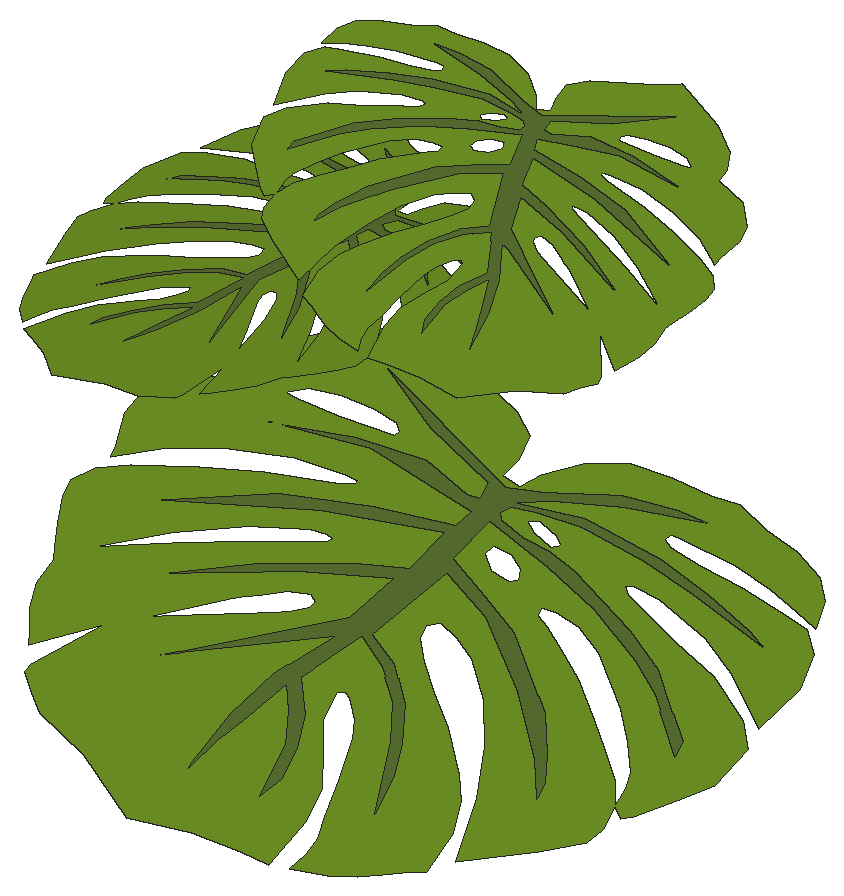
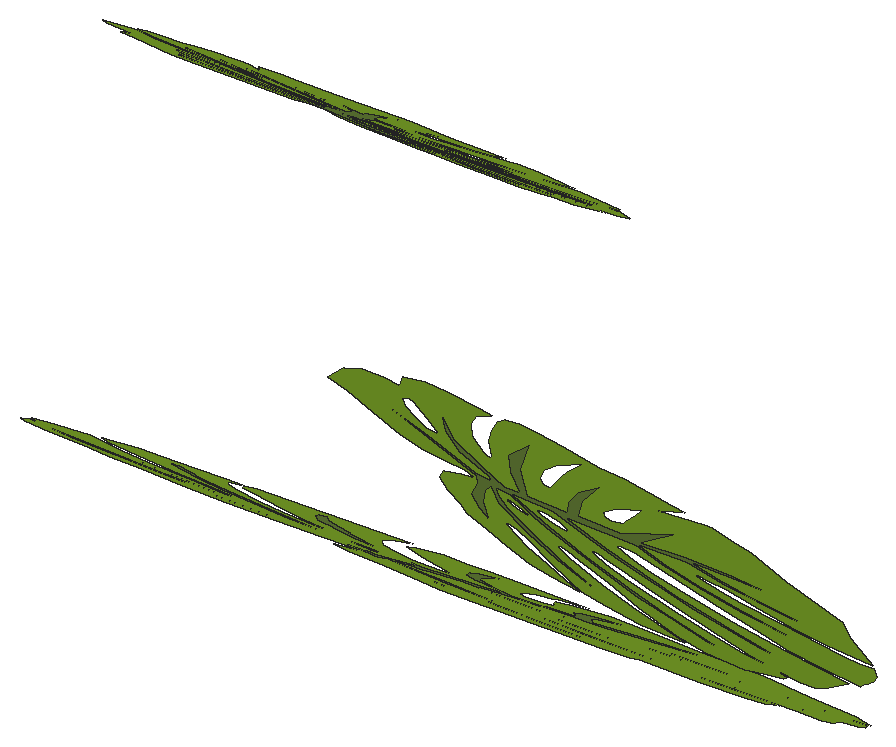
# SketchUp Ruby script. Lengths in inches.
U = 1.inch
M = Sketchup.active_model
def pt(a) = Geom::Point3d.new(a.map { |v| v * U })
def face(e, loops, mat)
  f = e.add_face(loops[0].map { |a| pt(a) })
  loops[1..].each { |l| e.add_face(l.map { |a| pt(a) }).erase! }
  f.material = f.back_material = mat if mat
  f
end
# faces: each face lists its corners as indices into pts; further lists are holes
def faces(e, pts, list, mat = nil) = list.each { |f| face(e, (f[0].is_a?(Array) ? f : [f]).map { |l| l.map { |i| pts[i] } }, mat) }
# xy, xz, yz: faces in a plane at the given z, y or x. An outline is a flat list of corners, or four numbers for a rectangle; further outlines are holes
def ring(l) = l.size == 4 ? [[l[0], l[1]], [l[2], l[1]], [l[2], l[3]], [l[0], l[3]]] : l.each_slice(2).to_a
def flat(e, list, mat, &to3) = list.each { |f| face(e, (f[0].is_a?(Array) ? f : [f]).map { |l| ring(l).map { |u, v| to3.(u, v) } }, mat) }
def xy(e, z, list, mat = nil) = flat(e, list, mat) { |x, y| [x, y, z] }
def xz(e, y, list, mat = nil) = flat(e, list, mat) { |x, z| [x, y, z] }
def yz(e, x, list, mat = nil) = flat(e, list, mat) { |y, z| [x, y, z] }
def lines(e, pts, list) = list.each { |a, b| e.add_line(pt(pts[a]), pt(pts[b])) }
# prism: a flat outline (further loops are holes) pulled along v
def prism(e, loops, v, mat = nil)
  f = face(e, loops, mat); d = Geom::Vector3d.new(v.map { |x| x * U })
  f.pushpull(f.normal.samedirection?(d) ? d.length : -d.length)
end
def box(e, o, s, mat = nil) = prism(e, [[o, [o[0] + s[0], o[1], o[2]], [o[0] + s[0], o[1] + s[1], o[2]], [o[0], o[1] + s[1], o[2]]]], [0, 0, s[2]], mat)
def at(x, y, z, deg = 0) = Geom::Transformation.translation(pt([x, y, z])) * Geom::Transformation.rotation(ORIGIN, Z_AXIS, deg.degrees)
def axes(o, x, y, z) = Geom::Transformation.new([*x, 0, *y, 0, *z, 0, *pt(o).to_a, 1])
def part(name) = M.definitions.add(name)
# library, detail: a bought-in or finely detailed component or shape, given as its bounding box
def library(name, o, s) = part(name).tap { |d| box(d.entities, o, s) }
def detail(e, o, s) = box(e.add_group.entities, o, s)
def put(e, d, t, mat = nil) = e.add_instance(d, t).tap { |i| i.material = mat if mat }
def group(e, t, mat = nil) = e.add_group.tap { |g| g.transformation = t; g.material = mat if mat }.entities
root = M.entities
M.materials.add("[0059_DarkOliveGreen]").color = [85, 107, 47]
M.materials.add("[0061_OliveDrab]").color = [107, 142, 35]
p = [[520.239,153.728,22.334],[520.977,153.593,22.249],[521.408,154.12,22.583],[522.47,154.844,23.043],[523.928,155.29,23.326],[525.483,155.364,23.372],
  [527.043,155.298,23.331],[528.141,155.35,23.364],[529.435,154.984,23.132],[530.862,154.714,22.96],[532.104,154.265,22.675],[532.723,153.723,22.331],
  [533.025,152.934,21.83],[532.093,153.181,21.987],[530.828,153.488,22.182],[529.252,153.745,22.345],[527.011,153.899,22.443],[526.638,153.881,22.431],
  [526.532,153.708,22.322],[526.902,153.559,22.227],[528.159,153.379,22.113],[529.904,153.234,22.021],[532.065,152.927,21.826],[532.759,152.811,21.753],
  [533.5,152.24,21.39],[533.766,151.206,20.734],[533.323,149.779,19.828],[531.296,150.951,20.572],[529.832,151.573,20.967],[527.617,152.106,21.305],
  [526.505,152.213,21.373],[526.248,152.109,21.307],[526.529,151.906,21.178],[527.285,151.694,21.044],[528.944,151.172,20.712],[530.863,150.663,20.389],
  [532.636,149.846,19.871],[533.406,149.141,19.423],[533.12,147.885,18.626],[532.28,147.119,18.14],[531.289,146.285,17.61],[530.906,146.106,17.497],
  [530.469,146.351,17.652],[530.45,146.926,18.017],[530.274,147.368,18.298],[529.562,148.138,18.787],[528.645,148.933,19.291],[526.842,150.145,20.06],
  [525.69,150.597,20.347],[524.704,150.736,20.435],[524.157,150.71,20.419],[524.197,150.465,20.263],[524.687,150.278,20.145],[525.582,149.835,19.864],
  [526.719,149.264,19.502],[528.052,148.375,18.937],[528.935,147.761,18.547],[529.953,147.029,18.083],[530.587,145.623,17.19],[530.336,145.135,16.881],
  [529.048,144.431,16.434],[526.716,143.335,15.738],[526.091,145.152,16.891],[525.239,146.591,17.805],[524.247,147.765,18.55],[523.042,148.695,19.14],
  [522.129,149.096,19.394],[521.358,149.33,19.543],[520.964,149.078,19.383],[521.028,148.686,19.134],[521.632,148.134,18.784],[522.555,147.456,18.354],
  [523.711,146.693,17.869],[525.038,145.584,17.166],[525.645,144.928,16.749],[526.0625,144.019,16.173],[526.027,142.793,15.394],[525.311,142.526,15.225],
  [524.754,142.268,15.061],[524,141.974,14.875],[523.069,141.698,14.7],[521.757,141.5,14.574],[521.958,141.994,14.888],[522.013,142.537,15.232],
  [521.76,143.172,15.635],[521.467,144.232,16.308],[521.038,145.456,17.084],[520.687,145.968,17.409],[520.114,146.479,17.734],[519.797,146.582,17.799],
  [519.588,146.465,17.725],[519.651,146.076,17.478],[519.728,145.601,17.176],[520.331,144.878,16.718],[521.117,143.818,16.045],[521.274,142.853,15.432],
  [521.048,141.374,14.494],[519.906,141.415,14.52],[518.002,141.406,14.514],[515.688,141.161,14.358],[513.072,142.342,15.108],[510.856,142.96,15.5],
  [510.215,143.416,15.79],[509.573,143.871,16.079],[509.617,144.147,16.254],[511.051,145.867,17.346],[509.885,145.112,16.866],[509.122,144.609,16.547],
  [508.903,144.952,16.765],[508.417,145.561,17.151],[508.134,146.268,17.6],[508.149,147.035,18.087],[507.939,147.365,18.296],[507.535,148.016,18.709],
  [507.135,148.747,19.173],[507.041,149.268,19.504],[507.566,149.822,19.855],[508.582,150.238,20.119],[510.698,150.89,20.533],[512.804,151.417,20.868],
  [515.421,151.879,21.161],[515.892,152.019,21.249],[515.876,152.12,21.314],[515.397,152.167,21.344],[513.461,152.076,21.286],[511.296,151.658,21.02],
  [509.326,151.059,20.64],[507.788,150.253,20.129],[507.731,150.604,20.352],[507.321,151.534,20.942],[507.475,152.24,21.39],[508.405,153.114,21.944],
  [510.241,153.597,22.251],[510.156,154.121,22.584],[510.574,154.859,23.052],[512.01,155.715,23.595],[514.962,156.822,24.298],[515.988,156.441,24.056],
  [517.607,155.999,23.776],[519.337,155.496,23.457],[520.273,155.004,23.144],[520.39,154.282,22.686],[518.431,148.552,19.049],[513.403,145.677,17.225],
  [518.35,147.893,18.631],[517.287,146.364,17.661],[516.782,144.862,16.707],[516.578,143.22,15.666],[516.566,143.072,15.571],[516.917,144.063,16.2],
  [517.257,144.808,16.673],[517.863,146.206,17.561],[518.468,145.532,17.133],[519.09,144.616,16.551],[519.342,143.064,15.566],[519.667,143.697,15.968],
  [519.517,144.624,16.556],[519.048,145.592,17.171],[518.197,146.488,17.739],[519.216,148.156,18.798],[520.445,147.601,18.446],[521.489,146.808,17.943],
  [522.275,145.764,17.28],[523.251,143.743,15.997],[523.066,144.883,16.721],[522.672,145.793,17.299],[521.912,146.866,17.98],[520.801,147.799,18.571],
  [519.496,148.335,18.911],[520.527,150.634,20.37],[522.592,149.906,19.909],[525.25,148.244,18.854],[527.034,146.778,17.923],[527.919,145.773,17.285],
  [527.845,146.229,17.575],[527.318,146.995,18.061],[526.387,148.058,18.736],[523.821,149.814,19.85],[522.208,150.444,20.25],[520.453,151.089,20.659],
  [520.797,152.4,21.491],[523.497,151.81,21.117],[525.806,151.181,20.718],[528.099,150.283,20.148],[529.398,149.627,19.732],[531.307,148.244,18.854],
  [531.235,148.688,19.135],[530.237,149.4,19.588],[529.041,150.3,20.159],[527.361,151.03,20.622],[524.41,151.986,21.228],[523.279,152.252,21.397],
  [522.101,152.349,21.459],[521.116,152.555,21.59],[520.9375,152.74,21.707],[521.184,152.971,21.854],[522.031,153.084,21.926],[523.749,153.165,21.977],
  [526.337,152.908,21.814],[528.506,152.571,21.6],[531.943,151.882,21.162],[531.023,152.218,21.376],[528.97,152.759,21.72],[526.8,153.184,21.989],
  [523.632,153.454,22.16],[521.277,153.163,21.976],[522.379,153.559,22.227],[524.638,154.099,22.57],[527.701,154.565,22.865],[526.307,154.596,22.885],
  [524.315,154.412,22.769],[521.829,153.719,22.329],[520.565,153.457,22.162],[514.225,155.41,23.402],[517.013,154.195,22.631],[519.922,153.378,22.112],
  [519.998,152.906,21.8125],[519.516,152.883,21.798],[517.587,153.351,22.095],[514.937,153.226,22.015],[511.951,152.729,21.7],[515.647,153.069,21.916],
  [518.13,152.723,21.696],[520.003,152.467,21.534],[519.793,151.994,21.234],[516.853,151.63,21.003],[513.708,151.027,20.62],[509.929,149.559,19.688],
  [515.374,150.972,20.585],[519.597,151.665,21.025],[519.278,150.415,20.231],[517.501,149.997,19.967],[514.48,149.005,19.337],[511.591,147.71,18.515],
  [515.962,149.211,19.467],[518.978,149.955,19.94],[513.428,149.857,19.877],[512.041,149.289,19.517],[511.268,148.972,19.316],[508.928,147.683,18.498],
  [509.849,148.025,18.715],[511.774,148.772,19.189],[513.71,149.419,19.6],[515.474,150,19.968],[516.209,150.245,20.124],[516.298,150.385,20.213],
  [516.027,150.448,20.253],[515.398,150.397,20.22],[515.212,148.223,18.841],[514.812,148.039,18.724],[514.426,147.862,18.611],[512.179,146.515,17.757],
  [514.023,147.177,18.177],[516.004,147.898,18.634],[516.507,148.072,18.745],[516.998,148.382,18.941],[517.074,148.601,19.08],[516.762,148.742,19.17],
  [515.998,148.585,19.07],[514.252,154.151,22.603],[513.588,154.164,22.611],[512.464,154.008,22.512],[511.82,153.664,22.294],[512.246,153.608,22.258],
  [514.006,153.588,22.245],[516.113,153.638,22.277],[516.179,153.794,22.376],[515.888,153.999,22.507],[514.916,154.137,22.594],[521.268,151.538,20.944],
  [521.805,151.154,20.701],[522.596,151.038,20.627],[522.907,151.174,20.713],[522.71,151.51,20.926],[522.132,151.777,21.096],[521.398,151.832,21.131],
  [522.852,152.786,21.736],[522.311,152.913,21.817],[521.917,152.787,21.737],[522.368,152.557,21.591],[523.188,152.358,21.465],[523.484,152.509,21.56],
  [523.074,152.733,21.703],[518.622,156.433,29.335],[519.41,156.337,29.494],[519.887,155.03,29.031],[519.861,154.246,28.672],[519.455,153.79,28.363],
  [518.989,153.568,28.144],[519.453,152.851,27.941],[519.176,152.194,27.575],[518.673,151.824,27.28],[517.725,151.5,26.89],[517.413,151.351,26.743],
  [517.351,152.139,27.081],[516.919,152.946,27.332],[516.249,153.72,27.507],[515.42,154.281,27.545],[515.157,154.387,27.525],[515.067,154.344,27.483],
  [515.174,154.152,27.424],[516.019,153.237,27.231],[516.573,152.427,27.01],[517.03,151.556,26.737],[517.165,151.09,26.5625],[516.96,150.691,26.331],
  [516.492,150.473,26.112],[515.71,150.239,25.806],[514.992,150.044,25.534],[514.626,149.946,25.395],[514.008,149.583,25.074],[513.301,149.33,24.778],
  [512.579,149.175,24.523],[512.198,149.074,24.379],[512.251,149.513,24.59],[512.321,150.178,24.906],[511.59,148.991,24.186],[511.386,148.85,24.07],
  [510.716,148.809,23.879],[510.046,148.768,23.688],[508.51,149.073,23.43],[506.327,149.222,22.935],[505.447,149.956,23.038],[504.565,150.469,23.041],
  [503.999,150.756,23.024],[505.097,151.507,23.643],[505.956,151.915,24.048],[507.185,152.199,24.492],[508.055,152.375,24.794],[508.477,152.577,24.993],
  [508.823,152.741,25.156],[508.821,152.852,25.206],[508.589,152.889,25.162],[507.906,152.803,24.948],[507.326,152.658,24.734],[506.13,152.202,24.221],
  [505.13,151.786,23.777],[504.495,151.557,23.511],[504.079,151.289,23.284],[503.771,151.005,23.077],[503.32,151.448,23.16],[503.11,151.827,23.275],
  [502.997,152.165,23.398],[502.946,152.435,23.506],[502.83,152.751,23.618],[503.811,153.333,24.132],[504.746,153.645,24.513],[505.563,153.789,24.787],
  [507.085,153.951,25.252],[508.245,153.998,25.572],[509.227,154.067,25.855],[509.959,154.163,26.087],[510.307,154.329,26.251],[510.329,154.552,26.357],
  [509.778,154.649,26.258],[509.026,154.706,26.09],[507.707,154.595,25.701],[506.289,154.313,25.209],[504.72,153.869,24.606],[502.949,153.188,23.845],
  [502.753,154.324,24.304],[502.725,154.997,24.599],[503.004,155.292,24.804],[503.652,155.6,25.109],[504.445,155.779,25.393],[505.516,155.848,25.699],
  [506.427,155.898,25.957],[507.773,155.956,26.329],[508.768,155.919,26.568],[509.547,155.885,26.754],[509.927,155.842,26.832],[510.145,155.945,26.935],
  [509.911,156.104,26.945],[509.338,156.303,26.887],[508.432,156.4,26.698],[506.605,156.317,26.19],[505.53,156.192,25.857],[504.571,156.023,25.535],
  [504.129,155.863,25.349],[503.249,155.603,25.006],[503.216,155.789,25.081],[503.433,156.444,25.431],[503.663,157.026,25.751],[504.552,157.688,26.277],
  [505.485,157.811,26.573],[506.977,157.718,26.915],[508.288,157.442,27.128],[509.487,157.242,27.347],[510.012,157.138,27.435],[510.308,157.158,27.52],
  [510.273,157.275,27.564],[509.666,157.523,27.519],[508.199,157.867,27.296],[507.01,157.969,27.036],[505.11,157.964,26.544],[506.065,158.749,27.142],
  [507.03,159.16,27.576],[507.841,159.228,27.815],[508.259,159.096,27.863],[509.518,158.662,27.992],[510.449,158.262,28.052],[511.183,158.01,28.128],
  [511.477,157.98,28.19],[511.568,158.089,28.263],[511.408,158.197,28.27],[510.237,158.725,28.206],[509.293,159.027,28.098],[508.453,159.223,27.97],
  [507.816,159.356,27.866],[508.599,159.644,28.196],[509.33,159.731,28.424],[510.275,159.608,28.612],[511.16,159.353,28.725],[512.062,159.177,28.878],
  [512.532,158.859,28.856],[513.313,158.472,28.884],[513.979,158.022,28.853],[514.297,157.423,28.666],[514.203,156.801,28.363],[513.975,156.44,28.142],
  [514.429,156.305,28.199],[514.811,156.604,28.431],[515.452,156.91,28.733],[516.29,156.889,28.939],[517.506,156.66,29.15],[516.315,155.66,28.394],
  [518.605,155.481,28.903],[517.134,155.734,28.639],[514.057,156.266,28.085],[513.681,156.726,28.195],[513.085,157.715,28.485],[512.304,158.334,28.562],
  [511.628,158.693,28.549],[512.679,157.656,28.354],[513.293,156.799,28.128],[513.486,156.319,27.962],[512.623,157.085,28.084],[510.925,157.807,27.971],
  [509.567,158.19,27.793],[508.168,158.487,27.566],[507.465,158.576,27.425],[509.63,157.978,27.714],[510.917,157.555,27.855],[512.334,156.982,27.963],
  [513.07,156.484,27.929],[513.373,156.205,27.882],[513.3,156.031,27.785],[513.066,155.993,27.708],[512.439,156.16,27.621],[511.81,156.43,27.58],
  [511.065,156.608,27.469],[508.911,156.952,27.069],[507.532,157.061,26.763],[506.242,156.961,26.386],[505.197,156.896,26.087],[504.801,156.708,25.901],
  [506.818,156.843,26.481],[507.958,156.801,26.756],[509.759,156.606,27.132],[511.349,156.282,27.395],[513.089,155.835,27.642],[512.182,155.131,27.093],
  [510.838,155.299,26.823],[509.573,155.437,26.559],[506.947,155.305,25.824],[505.647,155.058,25.379],[504.778,154.841,25.058],[504.372,154.648,24.866],
  [505.603,154.88,25.287],[507.628,155.087,25.902],[510.222,155.151,26.598],[511.777,154.938,26.903],[510.388,153.589,25.94],[509.342,153.688,25.715],
  [508.065,153.55,25.325],[506.837,153.253,24.875],[505.912,152.934,24.494],[504.898,152.451,24.016],[506.999,153.133,24.863],[508.215,153.41,25.3],
  [509.348,153.501,25.632],[510.373,153.431,25.865],[509.491,152.38,25.166],[508.364,152.189,24.791],[507.358,151.863,24.385],[506.534,151.471,23.997],
  [506.17,151.088,23.732],[507.551,151.745,24.382],[508.586,152.006,24.766],[509.417,152.159,25.048],[508.5625,151.344,24.462],[508.115,150.905,24.15],
  [507.472,150.349,23.735],[507.588,150.421,23.797],[508.828,151.242,24.485],[509.815,152.078,25.114],[510.563,153.076,25.754],[511.068,150.718,24.826],
  [511.062,153.405,26.031],[511.948,154.207,26.618],[512.75,153.052,26.306],[513.569,151.182,25.678],[513.274,152.56,26.221],[512.672,153.831,26.636],
  [512.182,154.502,26.811],[513.051,155.17,27.334],[514.458,153.717,27.044],[515.849,151.6,26.452],[515.279,153.297,27.067],[514.303,154.42,27.32],
  [513.227,155.376,27.472],[513.514,155.653,27.67],[514.596,155.272,27.778],[516.037,154.768,27.923],[517.485,153.62,27.78],[516.495,154.652,27.988],
  [515.36,155.419,28.041],[514.08,155.717,27.845],[513.873,155.857,27.854],[514.293,156.057,28.052],[514.458,152.675,26.577],[513.978,153.455,26.803],
  [513.726,153.647,26.825],[513.549,153.69,26.799],[513.477,153.601,26.74],[513.62,153.29,26.637],[513.97,152.547,26.394],[514.347,151.726,26.123],
  [514.638,150.863,25.81],[514.789,150.457,25.667],[514.746,151.685,26.207],[512.224,152.77,26.044],[511.995,153.047,26.11],[511.735,153.065,26.051],
  [511.592,152.942,25.959],[511.569,152.667,25.83],[511.662,152.451,25.757],[512,151.584,25.455],[512.322,150.782,25.177],[512.369,152.012,25.741],
  [517.889,154.729,28.381],[517.247,155.071,28.37],[516.681,155.267,28.3125],[516.378,155.249,28.226],[516.282,155.159,28.161],[517.225,154.572,28.14],
  [518.0625,154.11,28.148],[518.307,154.022,28.172],[518.286,154.355,28.316],[511.958,155.901,27.381],[511.472,155.931,27.27],[511.106,155.827,27.129],
  [511.14,155.68,27.072],[511.604,155.523,27.12],[512.167,155.558,27.281],[512.346,155.73,27.404],[512.8,156.479,27.857],[512.297,156.6,27.782],
  [511.923,156.605,27.688],[511.939,156.455,27.625],[512.483,156.328,27.708],[512.88,156.315,27.804],[522.447,153.259,35.965],[521.96,153.17,35.909],
  [521.675,153.517,36.129],[520.974,153.996,36.433],[520.012,154.29,36.62],[518.986,154.338,36.65],[517.956,154.295,36.623],[517.232,154.329,36.645],
  [516.377,154.088,36.491],[515.436,153.91,36.378],[514.616,153.613,36.19],[514.207,153.255,35.963],[514.008,152.734,35.632],[514.623,152.898,35.736],
  [515.458,153.1,35.865],[516.498,153.27,35.972],[517.977,153.371,36.037],[518.224,153.36,36.029],[518.293,153.245,35.957],[518.049,153.147,35.895],
  [517.22,153.028,35.819],[516.068,152.933,35.759],[514.642,152.73,35.63],[514.184,152.654,35.581],[513.694,152.277,35.342],[513.519,151.594,34.909],
  [513.812,150.652,34.311],[515.149,151.426,34.802],[516.115,151.836,35.0625],[517.577,152.188,35.286],[518.311,152.259,35.331],[518.481,152.19,35.287],
  [518.296,152.056,35.202],[517.797,151.917,35.113],[516.702,151.572,34.895],[515.435,151.236,34.681],[514.265,150.697,34.339],[513.757,150.231,34.044],
  [513.945,149.402,33.518],[514.5,148.897,33.197],[515.154,148.346,32.847],[515.407,148.228,32.773],[515.695,148.39,32.875],[515.708,148.769,33.116],
  [515.823,149.061,33.301],[516.294,149.57,33.624],[516.899,150.094,33.957],[518.089,150.894,34.464],[518.849,151.192,34.654],[519.5,151.284,34.712],
  [519.861,151.267,34.701],[519.834,151.105,34.598],[519.511,150.982,34.52],[518.92,150.69,34.335],[518.17,150.313,34.096],[517.29,149.726,33.723],
  [516.707,149.321,33.466],[516.036,148.837,33.159],[515.617,147.909,32.57],[515.783,147.587,32.366],[516.633,147.123,32.071],[518.172,146.399,31.612],
  [518.584,147.599,32.373],[519.147,148.548,32.976],[519.802,149.323,33.468],[520.597,149.937,33.857],[521.199,150.201,34.025],[521.708,150.356,34.123],
  [521.968,150.189,34.017],[521.926,149.931,33.853],[521.528,149.567,33.622],[520.918,149.12,33.338],[520.156,148.616,33.018],[519.28,147.884,32.554],
  [518.879,147.451,32.279],[518.603,146.851,31.899],[518.627,146.041,31.385],[519.099,145.865,31.273],[519.467,145.695,31.165],[519.964,145.501,31.042],
  [520.579,145.319,30.926],[521.445,145.188,30.843],[521.312,145.514,31.05],[521.276,145.873,31.278],[521.443,146.292,31.544],[521.637,146.992,31.988],
  [521.92,147.799,32.5],[522.151,148.137,32.715],[522.529,148.474,32.929],[522.738,148.543,32.972],[522.877,148.465,32.923],[522.835,148.208,32.76],
  [522.784,147.895,32.561],[522.386,147.418,32.258],[521.867,146.718,31.814],[521.764,146.081,31.41],[521.913,145.105,30.79],[522.667,145.132,30.808],
  [523.923,145.127,30.804],[525.45,144.964,30.701],[527.177,145.744,31.196],[528.64,146.152,31.455],[529.063,146.453,31.646],[529.486,146.753,31.837],
  [529.457,146.936,31.952],[528.511,148.071,32.673],[529.281,147.572,32.356],[529.784,147.241,32.146],[529.929,147.467,32.289],[530.249,147.869,32.544],
  [530.436,148.335,32.84],[530.426,148.842,33.162],[530.565,149.059,33.3],[530.831,149.489,33.573],[531.096,149.971,33.879],[531.158,150.315,34.097],
  [530.811,150.681,34.329],[530.141,150.955,34.503],[528.744,151.386,34.776],[527.354,151.733,34.997],[525.627,152.038,35.191],[525.316,152.13,35.249],
  [525.327,152.197,35.292],[525.643,152.229,35.312],[526.92,152.169,35.273],[528.349,151.892,35.098],[529.65,151.497,34.847],[530.665,150.965,34.51],
  [530.702,151.197,34.657],[530.972,151.811,35.046],[530.871,152.277,35.342],[530.257,152.853,35.708],[529.045,153.172,35.91],[529.101,153.518,36.13],
  [528.826,154.005,36.439],[527.878,154.57,36.797],[525.929,155.3,37.261],[525.253,155.049,37.102],[524.184,154.758,36.916],[523.042,154.426,36.706],
  [522.425,154.101,36.5],[522.347,153.625,36.197],[523.64,149.843,33.797],[526.959,147.945,32.593],[523.693,149.408,33.521],[524.395,148.399,32.881],
  [524.728,147.407,32.251],[524.863,146.324,31.564],[524.871,146.226,31.502],[524.639,146.88,31.917],[524.415,147.371,32.229],[524.015,148.294,32.815],
  [523.615,147.849,32.532],[523.205,147.245,32.148],[523.039,146.22,31.498],[522.824,146.638,31.764],[522.923,147.25,32.152],[523.233,147.889,32.557],
  [523.794,148.48,32.933],[523.122,149.581,33.631],[522.311,149.215,33.399],[521.622,148.692,33.067],[521.103,148.003,32.63],[520.459,146.668,31.783],
  [520.581,147.421,32.26],[520.841,148.022,32.642],[521.343,148.73,33.091],[522.076,149.345,33.482],[522.937,149.699,33.706],[522.257,151.216,34.669],
  [520.894,150.737,34.365],[519.139,149.639,33.668],[517.962,148.672,33.054],[517.378,148.008,32.633],[517.427,148.31,32.824],[517.775,148.815,33.145],
  [518.389,149.517,33.59],[520.083,150.675,34.326],[521.147,151.091,34.59],[522.305,151.517,34.86],[522.079,152.382,35.409],[520.296,151.993,35.162],
  [518.773,151.578,34.898],[517.259,150.985,34.522],[516.402,150.552,34.248],[515.142,149.639,33.668],[515.19,149.932,33.854],[515.848,150.402,34.152],
  [516.637,150.996,34.529],[517.747,151.478,34.835],[519.694,152.109,35.235],[520.44,152.284,35.347],[521.218,152.349,35.388],[521.868,152.485,35.474],
  [521.986,152.607,35.551],[521.823,152.759,35.648],[521.264,152.834,35.696],[520.13,152.887,35.73],[518.422,152.718,35.622],[516.991,152.495,35.481],
  [514.722,152.04,35.192],[515.329,152.262,35.333],[516.685,152.619,35.56],[518.117,152.9,35.738],[520.207,153.078,35.85],[521.762,152.886,35.729],
  [521.034,153.147,35.894],[519.543,153.504,36.121],[517.522,153.811,36.316],[518.442,153.832,36.329],[519.757,153.71,36.252],[521.398,153.253,35.961],
  [522.232,153.08,35.852],[526.416,154.369,36.67],[524.576,153.567,36.161],[522.656,153.027,35.818],[522.606,152.716,35.621],[522.924,152.701,35.611],
  [524.197,153.01,35.807],[525.946,152.927,35.755],[527.917,152.599,35.547],[525.478,152.824,35.689],[523.839,152.595,35.544],[522.602,152.426,35.437],
  [522.741,152.114,35.239],[524.682,151.874,35.087],[526.757,151.476,34.834],[529.252,150.507,34.219],[525.658,151.44,34.811],[522.871,151.897,35.101],
  [523.081,151.072,34.577],[524.254,150.797,34.403],[526.248,150.142,33.987],[528.155,149.287,33.445],[525.269,150.277,34.073],[523.279,150.769,34.385],
  [526.942,150.704,34.344],[527.858,150.329,34.106],[528.368,150.12,33.973],[529.912,149.269,33.433],[529.304,149.495,33.577],[528.034,149.988,33.889],
  [526.756,150.415,34.16],[525.592,150.798,34.404],[525.107,150.96,34.506],[525.048,151.053,34.565],[525.227,151.094,34.591],[525.642,151.06,34.57],
  [525.765,149.626,33.66],[526.029,149.504,33.582],[526.283,149.387,33.508],[527.766,148.498,32.944],[526.549,148.935,33.221],[525.242,149.411,33.523],
  [524.91,149.526,33.596],[524.586,149.73,33.726],[524.536,149.875,33.818],[524.742,149.968,33.877],[525.246,149.864,33.811],[526.398,153.538,36.142],
  [526.837,153.547,36.148],[527.578,153.444,36.083],[528.003,153.217,35.939],[527.722,153.18,35.915],[526.561,153.166,35.907],[525.17,153.199,35.928],
  [525.126,153.302,35.993],[525.319,153.438,36.079],[525.96,153.529,36.137],[521.768,151.813,35.048],[521.413,151.56,34.887],[520.891,151.483,34.838],
  [520.686,151.573,34.895],[520.816,151.795,35.036],[521.198,151.971,35.148],[521.682,152.007,35.171],[520.722,152.637,35.571],[521.08,152.721,35.624],
  [521.339,152.637,35.571],[521.041,152.486,35.475],[520.5,152.355,35.391],[520.305,152.454,35.454],[520.576,152.602,35.549],[522.715,151.507,20.925],
  [520.813,151.793,35.035]]
faces(root,p,[[[0,1,2,3,4,5,6,7,8,9,10,11,12,13,14,15,16,17,18,19,20,21,22,23,24,25,26,27,28,29,30,31,32,33,34,35,36,37,38,39,40,41,42,43,44,45,46,47,48,49,50,51,52,53,54,55,56,57,42,58,59,60,61,62,63,64,65,66,67,68,69,70,71,72,73,74,75,76,77,78,79,80,81,82,83,84,85,86,87,88,89,90,91,92,93,94,95,96,97,98,99,100,101,102,103,104,105,106,107,108,109,110,111,112,113,114,115,116,117,118,119,120,121,122,123,124,125,126,127,128,129,130,131,132,133,134,135,136,137,138,139,140,141],[142,143,144,145,146,147,148,149,150,151,152,153,154,155,156,157,158,159,160,161,162,163,164,165,166,167,168,169,170,171,172,173,174,175,176,177,178,179,180,181,182,183,184,185,186,187,188,189,190,191,192,193,194,195,196,197,198,199,200,201,202,203,204,205,206,207,208,209,210,211,212,213,214,215,216,217,218,219,220,221,222,223,224,225,226,227,228,229,230,231,232,233,234,235],[236,237,238,239,240,241,242,243,244,245,246,247],[248,249,250,251,252,253,254,255,256,257,258],[259,260,261,262,263,264,265,266,267,268],[269,270,271,272,273,274,275],[276,277,278,279,280,281,282]],[[283,284,285,286,287,288,289,290,291,292,293,294,295,296,297,298,299,300,301,302,303,304,305,306,307,308,309,310,311,312,313,314,315,316,317,318,319,320,321,322,323,324,325,326,327,328,329,330,331,332,333,334,335,336,337,338,339,340,341,342,343,344,345,346,347,348,349,350,351,352,353,354,355,356,357,358,359,360,361,362,363,364,365,366,367,368,369,370,371,372,373,374,375,376,377,378,363,379,380,381,382,383,384,385,386,387,388,389,390,391,392,393,394,395,396,397,398,399,400,401,402,403,404,405,406,407,408,409,410,411,412,413,414,415,416,417,418,419,420,421,422,423,424],[425,426,427,428,429,430,431,432,433,434,435,436,437,438,439,440,441,442,443,444,445,446,447,448,449,450,451,452,453,454,455,456,457,458,459,460,461,462,463,464,465,466,467,468,469,470,471,472,473,474,475,476,477,478,479,480,481,482,483,484,485,486,487,488,489,490,491,492,493,494,495,496,497,498,499,500,501,502,503,504,505,506,507,508,509,510,511,512,513,514,515,516,517,518,519],[520,521,522,523,524,525,526,527,528,529,530],[531,532,533,534,535,536,537,538,539],[540,541,542,543,544,545,546,547,548],[549,550,551,552,553,554,555],[556,557,558,559,560,561]],[[562,563,564,565,566,567,568,569,570,571,572,573,574,575,576,577,578,579,580,581,582,583,584,585,586,587,588,589,590,591,592,593,594,595,596,597,598,599,600,601,602,603,604,605,606,607,608,609,610,611,612,613,614,615,616,617,618,619,604,620,621,622,623,624,625,626,627,628,629,630,631,632,633,634,635,636,637,638,639,640,641,642,643,644,645,646,647,648,649,650,651,652,653,654,655,656,657,658,659,660,661,662,663,664,665,666,667,668,669,670,671,672,673,674,675,676,677,678,679,680,681,682,683,684,685,686,687,688,689,690,691,692,693,694,695,696,697,698,699,700,701,702,703],[704,705,706,707,708,709,710,711,712,713,714,715,716,717,718,719,720,721,722,723,724,725,726,727,728,729,730,731,732,733,734,735,736,737,738,739,740,741,742,743,744,745,746,747,748,749,750,751,752,753,754,755,756,757,758,759,760,761,762,763,764,765,766,767,768,769,770,771,772,773,774,775,776,777,778,779,780,781,782,783,784,785,786,787,788,789,790,791,792,793,794,795,796,797],[798,799,800,801,802,803,804,805,806,807,808,809],[810,811,812,813,814,815,816,817,818,819,820],[821,822,823,824,825,826,827,828,829,830],[831,832,833,834,835,836,837],[838,839,840,841,842,843,844]]],"[0061_OliveDrab]")
faces(root,p,[[143,142,235,234,233,232,231,230,229,228,227,226,225,224,223,222,221,220,219,218,217,216,215,214,213,212,211,210,209,208,207,206,205,204,203,202,201,200,199,198,197,196,195,194,193,192,191,190,189,188,187,186,185,184,183,182,181,180,179,178,177,176,175,174,173,172,171,170,169,168,167,166,165,164,163,162,161,160,159,158,157,156,155,154,153,152,151,150,149,148,147,146,145,144],[426,425,519,518,517,516,515,514,513,512,511,510,509,508,507,506,505,504,503,502,501,500,499,498,497,496,495,494,493,492,491,490,489,488,487,486,485,484,483,482,481,480,479,478,477,476,475,474,473,472,471,470,469,468,467,466,465,464,463,462,461,460,459,458,457,456,455,454,453,452,451,450,449,448,447,446,445,444,443,442,441,440,439,438,437,436,435,434,433,432,431,430,429,428,427],[705,704,797,796,795,794,793,792,791,790,789,788,787,786,785,784,783,782,781,780,779,778,777,776,775,774,773,772,771,770,769,768,767,766,765,764,763,762,761,760,759,758,757,756,755,754,753,752,751,750,749,748,747,746,745,744,743,742,741,740,739,738,737,736,735,734,733,732,731,730,729,728,727,726,725,724,723,722,721,720,719,718,717,716,715,714,713,712,711,710,709,708,707,706]],"[0059_DarkOliveGreen]")
lines(root,p,[[273,845],[835,846]])
